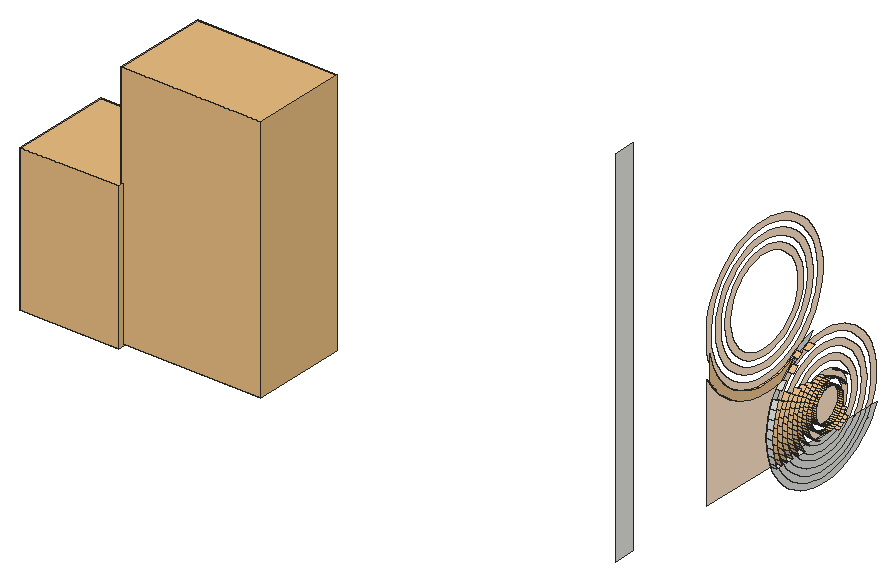
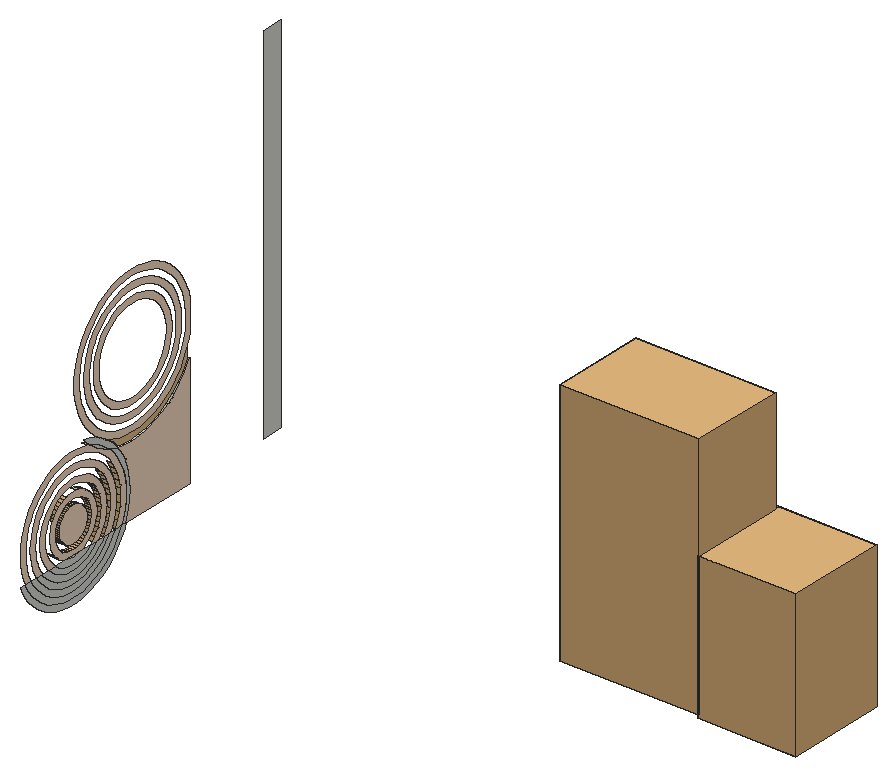
# SketchUp Ruby script. Lengths in inches.
U = 1.inch
M = Sketchup.active_model
def pt(a) = Geom::Point3d.new(a.map { |v| v * U })
def face(e, loops, mat)
  f = e.add_face(loops[0].map { |a| pt(a) })
  loops[1..].each { |l| e.add_face(l.map { |a| pt(a) }).erase! }
  f.material = f.back_material = mat if mat
  f
end
# faces: each face lists its corners as indices into pts; further lists are holes
def faces(e, pts, list, mat = nil) = list.each { |f| face(e, (f[0].is_a?(Array) ? f : [f]).map { |l| l.map { |i| pts[i] } }, mat) }
# xy, xz, yz: faces in a plane at the given z, y or x. An outline is a flat list of corners, or four numbers for a rectangle; further outlines are holes
def ring(l) = l.size == 4 ? [[l[0], l[1]], [l[2], l[1]], [l[2], l[3]], [l[0], l[3]]] : l.each_slice(2).to_a
def flat(e, list, mat, &to3) = list.each { |f| face(e, (f[0].is_a?(Array) ? f : [f]).map { |l| ring(l).map { |u, v| to3.(u, v) } }, mat) }
def xy(e, z, list, mat = nil) = flat(e, list, mat) { |x, y| [x, y, z] }
def xz(e, y, list, mat = nil) = flat(e, list, mat) { |x, z| [x, y, z] }
def yz(e, x, list, mat = nil) = flat(e, list, mat) { |y, z| [x, y, z] }
def lines(e, pts, list) = list.each { |a, b| e.add_line(pt(pts[a]), pt(pts[b])) }
# prism: a flat outline (further loops are holes) pulled along v
def prism(e, loops, v, mat = nil)
  f = face(e, loops, mat); d = Geom::Vector3d.new(v.map { |x| x * U })
  f.pushpull(f.normal.samedirection?(d) ? d.length : -d.length)
end
def box(e, o, s, mat = nil) = prism(e, [[o, [o[0] + s[0], o[1], o[2]], [o[0] + s[0], o[1] + s[1], o[2]], [o[0], o[1] + s[1], o[2]]]], [0, 0, s[2]], mat)
def at(x, y, z, deg = 0) = Geom::Transformation.translation(pt([x, y, z])) * Geom::Transformation.rotation(ORIGIN, Z_AXIS, deg.degrees)
def axes(o, x, y, z) = Geom::Transformation.new([*x, 0, *y, 0, *z, 0, *pt(o).to_a, 1])
def part(name) = M.definitions.add(name)
# library, detail: a bought-in or finely detailed component or shape, given as its bounding box
def library(name, o, s) = part(name).tap { |d| box(d.entities, o, s) }
def detail(e, o, s) = box(e.add_group.entities, o, s)
def put(e, d, t, mat = nil) = e.add_instance(d, t).tap { |i| i.material = mat if mat }
def group(e, t, mat = nil) = e.add_group.tap { |g| g.transformation = t; g.material = mat if mat }.entities
root = M.entities
M.materials.add("[Color C02]").color = [255, 228, 201]
M.materials.add("images").color = [235, 194, 141]
c1 = library("Group\#206",[0,0,0],[32.28,33.03,47.79])
c2 = library("Group\#215",[0,0,0],[15.67,22.625,14.53])
c3 = library("Group\#212",[0,0.16,0],[45.87,31.27,81.21])
xy(root,0,[[183.82,72.6875,185.82,74.8],[183.82,77.01,185.82,79.31],[183.82,81.7,185.82,84.26]])
xy(root,1.47,[[183.82,93.95,185.82,94.83]],"images")
xy(root,3.46,[[183.82,94.0625,185.82,94.72]],"images")
xy(root,14.7,[[183.82,94.0625,185.82,94.72]],"images")
xy(root,16.69,[[183.82,93.95,185.82,94.83]],"images")
yz(root,183.82,[[93.02,-14.45,95.76,-14.45,98.48,-14.125,101.15,-13.49,103.72,-12.56,106.17,-11.33,108.46,-9.82,110.5625,-8.0625,112.44,-6.07,114.08,-3.87,115.45,-1.5,116.09,0,113.98,0,113.71,-0.625,112.46,-2.8,110.96,-4.82,109.23,-6.65,107.3,-8.27,105.2,-9.65,102.96,-10.78,100.59,-11.64,98.14,-12.22,95.65,-12.51,93.13,-12.51,90.63,-12.22,88.1875,-11.64,85.82,-10.78,83.58,-9.65,81.48,-8.27,79.55,-6.65,77.82,-4.82,76.32,-2.8,75.06,-0.625,74.8,0,72.6875,0,73.33,-1.5,74.7,-3.87,76.34,-6.07,78.22,-8.0625,80.32,-9.82,82.61,-11.33,85.06,-12.56,87.63,-13.49,90.3,-14.125],[93.13,-12.51,95.65,-12.51,98.14,-12.22,100.59,-11.64,102.96,-10.78,105.2,-9.65,107.3,-8.27,109.23,-6.65,110.96,-4.82,112.46,-2.8,113.71,-0.625,113.98,0,111.77,0,110.79,-1.7,109.42,-3.53,107.86,-5.19,106.11,-6.66,104.2,-7.92,102.16,-8.94,100.02,-9.72,97.8,-10.25,95.53,-10.51,93.25,-10.51,90.98,-10.25,88.76,-9.72,86.62,-8.94,84.58,-7.92,82.67,-6.66,80.92,-5.19,79.36,-3.53,77.99,-1.7,77.01,0,74.8,0,75.06,-0.625,76.32,-2.8,77.82,-4.82,79.55,-6.65,81.48,-8.27,83.58,-9.65,85.82,-10.78,88.1875,-11.64,90.63,-12.22],[93.25,-10.51,95.53,-10.51,97.8,-10.25,100.02,-9.72,102.16,-8.94,104.2,-7.92,106.11,-6.66,107.86,-5.19,109.42,-3.53,110.79,-1.7,111.77,0,109.46,0,109.12,-0.61,107.89,-2.25,106.48,-3.74,104.91,-5.06,103.2,-6.18,101.37,-7.1,99.44,-7.8,97.45,-8.28,95.41,-8.52,93.36,-8.52,91.33,-8.28,89.33,-7.8,87.41,-7.1,85.58,-6.18,83.86,-5.06,82.29,-3.74,80.89,-2.25,79.66,-0.61,79.31,0,77.01,0,77.99,-1.7,79.36,-3.53,80.92,-5.19,82.67,-6.66,84.58,-7.92,86.62,-8.94,88.76,-9.72,90.98,-10.25],[93.36,-8.52,95.41,-8.52,97.45,-8.28,99.44,-7.8,101.37,-7.1,103.2,-6.18,104.91,-5.06,106.48,-3.74,107.89,-2.25,109.12,-0.61,109.46,0,107.08,0,106.36,-0.96,105.11,-2.29,103.72,-3.45,102.2,-4.45,100.58,-5.27,98.87,-5.89,97.1,-6.31,95.3,-6.52,93.48,-6.52,91.68,-6.31,89.91,-5.89,88.2,-5.27,86.58,-4.45,85.06,-3.45,83.67,-2.29,82.42,-0.96,81.7,0,79.31,0,79.66,-0.61,80.89,-2.25,82.29,-3.74,83.86,-5.06,85.58,-6.18,87.41,-7.1,89.33,-7.8,91.33,-8.28],[93.48,-6.52,95.3,-6.52,97.1,-6.31,98.87,-5.89,100.58,-5.27,102.2,-4.45,103.72,-3.45,105.11,-2.29,106.36,-0.96,107.08,0,104.52,0,103.74,-0.83,102.53,-1.85,101.2,-2.72,99.79,-3.43,98.3,-3.97,96.76,-4.34,95.18,-4.52,93.6,-4.52,92.02,-4.34,90.48,-3.97,88.99,-3.43,87.58,-2.72,86.25,-1.85,85.04,-0.83,84.26,0,81.7,0,82.42,-0.96,83.67,-2.29,85.06,-3.45,86.58,-4.45,88.2,-5.27,89.91,-5.89,91.68,-6.31],
  [93.6,-4.52,95.18,-4.52,96.76,-4.34,98.3,-3.97,99.79,-3.43,101.2,-2.72,102.53,-1.85,103.74,-0.83,104.52,0,101.625,0,101.33,-0.24,100.2,-0.99,98.99,-1.59,97.72,-2.06,96.41,-2.37,95.07,-2.53,93.71,-2.53,92.37,-2.37,91.06,-2.06,89.79,-1.59,88.58,-0.99,87.45,-0.24,87.16,0,84.26,0,85.04,-0.83,86.25,-1.85,87.58,-2.72,88.99,-3.43,90.48,-3.97,92.02,-4.34],[93.71,-2.53,95.07,-2.53,96.41,-2.37,97.72,-2.06,98.99,-1.59,100.2,-0.99,101.33,-0.24,101.625,0,97.54,0,97.15,-0.14,96.0625,-0.4,94.95,-0.53,93.83,-0.53,92.72,-0.4,91.63,-0.14,91.24,0,87.16,0,87.45,-0.24,88.58,-0.99,89.79,-1.59,91.06,-2.06,92.37,-2.37],[93.83,-0.53,94.95,-0.53,96.0625,-0.4,97.15,-0.14,97.54,0,91.24,0,91.63,-0.14,92.72,-0.4],[9,0,16,120],[72.6875,0,74.8,0,74.07,1.68,73.35,4.09,72.91,6.57,72.76,9.08,72.91,11.59,73.35,14.07,74.07,16.48,75.06,18.79,76.32,20.96,77.82,22.98,79.55,24.81,79.6,24.85,79.04,24.61,76.06,23.74,75.96,23.72,74.7,22.03,73.33,19.66,72.25,17.14,71.46,14.51,70.98,11.82,70.82,9.08,70.98,6.34,71.46,3.65,72.25,1.02],
  [75.96,23.72,76.06,23.74,79.04,24.61,79.6,24.85,81.48,26.43,83.58,27.81,85.82,28.9375,87.43,29.52,89.38,31.34,90.15,32.25,87.63,31.65,85.06,30.72,83.42,29.9,83.11,29.67,81.36,28.67,80.32,27.98,78.22,26.22,76.34,24.23],[79.6,24.85,81.9,25.83,84.6,27.37,87.11,29.22,87.43,29.52,85.82,28.9375,83.58,27.81,81.48,26.43],[81.36,28.67,83.11,29.67,83.42,29.9,82.61,29.49]])
yz(root,183.82,[[46.5625,0,72.6875,0,72.25,1.02,71.46,3.65,70.98,6.34,70.82,9.08,70.98,11.82,71.46,14.51,72.25,17.14,73.33,19.66,74.7,22.03,75.96,23.72,72.99,23.21,69.89,23.05,66.79,23.24,63.73,23.8,60.75,24.7,57.9,25.95,55.22,27.52,52.73,29.39,50.48,31.53,48.49,33.92,46.8,36.53,46.5625,37.01],[74.8,0,77.01,0,76.85,0.27,75.95,2.37,75.29,4.55,74.9,6.8,74.76,9.08,74.9,11.36,75.29,13.61,75.95,15.79,76.85,17.89,77.99,19.86,79.36,21.69,80.92,23.35,82.67,24.82,84.58,26.08,86.62,27.1,88.76,27.88,90.98,28.41,93.25,28.67,95.53,28.67,97.8,28.41,100.02,27.88,102.16,27.1,104.2,26.08,106.11,24.82,107.86,23.35,109.42,21.69,110.79,19.86,111.93,17.89,112.83,15.79,113.49,13.61,113.88,11.36,114.01,9.08,113.88,6.8,113.49,4.55,112.83,2.37,111.93,0.27,111.77,0,113.98,0,114.71,1.68,115.43,4.09,115.87,6.57,116.01,9.08,115.87,11.59,115.43,14.07,114.71,16.48,113.71,18.79,112.46,20.96,110.96,22.98,109.23,24.81,107.3,26.43,105.2,27.81,102.96,28.9375,100.59,29.8,98.14,30.375,95.65,30.67,93.13,30.67,90.63,30.375,88.1875,29.8,87.43,29.52,87.11,29.22,84.6,27.37,81.9,25.83,79.6,24.85,79.55,24.81,77.82,22.98,76.32,20.96,75.06,18.79,74.07,16.48,73.35,14.07,72.91,11.59,72.76,9.08,72.91,6.57,73.35,4.09,74.07,1.68],[79.31,0,81.7,0,81.34,0.49,80.43,2.07,79.71,3.74,79.1875,5.48,78.87,7.27,78.76,9.08,78.87,10.89,79.1875,12.68,79.71,14.42,80.43,16.09,81.34,17.67,82.42,19.125,83.67,20.45,85.06,21.61,86.58,22.61,88.2,23.43,89.91,24.05,91.68,24.47,93.48,24.68,95.3,24.68,97.1,24.47,98.87,24.05,100.58,23.43,102.2,22.61,103.72,21.61,105.11,20.45,106.36,19.125,107.44,17.67,108.35,16.09,109.07,14.42,109.59,12.68,109.91,10.89,110.01,9.08,109.91,7.27,109.59,5.48,109.07,3.74,108.35,2.07,107.44,0.49,107.08,0,109.46,0,110.14,1.17,110.95,3.05,111.54,5.02,111.9,7.03,112.01,9.08,111.9,11.125,111.54,13.14,110.95,15.11,110.14,16.99,109.12,18.77,107.89,20.41,106.48,21.9,104.91,23.22,103.2,24.34,101.37,25.26,99.44,25.96,97.45,26.4375,95.41,26.68,93.36,26.68,91.33,26.4375,89.33,25.96,87.41,25.26,85.58,24.34,83.86,23.22,82.29,21.9,80.89,20.41,79.66,18.77,78.64,16.99,77.83,15.11,77.24,13.14,76.88,11.125,76.76,9.08,76.88,7.03,77.24,5.02,77.83,3.05,78.64,1.17],[84.26,0,87.16,0,86.41,0.625,85.48,1.61,84.68,2.69,84,3.86,83.47,5.1,83.08,6.4,82.84,7.73,82.76,9.08,82.84,10.43,83.08,11.76,83.47,13.06,84,14.3,84.68,15.47,85.48,16.55,86.41,17.54,87.45,18.4,88.58,19.15,89.79,19.75,91.06,20.22,92.37,20.53,93.71,20.69,95.07,20.69,96.41,20.53,97.72,20.22,98.99,19.75,100.2,19.15,101.33,18.4,102.37,17.54,103.3,16.55,104.1,15.47,104.78,14.3,105.3125,13.06,105.7,11.76,105.9375,10.43,106.01,9.08,105.9375,7.73,105.7,6.4,105.3125,5.1,104.78,3.86,104.1,2.69,103.3,1.61,102.37,0.625,101.625,0,104.52,0,104.83,0.32,105.77,1.59,106.57,2.97,107.19,4.42,107.65,5.9375,107.92,7.5,108.01,9.08,107.92,10.66,107.65,12.22,107.19,13.74,106.57,15.19,105.77,16.57,104.83,17.84,103.74,18.99,102.53,20.01,101.2,20.88,99.79,21.59,98.3,22.13,96.76,22.5,95.18,22.68,93.6,22.68,92.02,22.5,90.48,22.13,88.99,21.59,87.58,20.88,86.25,20.01,85.04,18.99,83.95,17.84,83.01,16.57,82.21,15.19,81.59,13.74,81.13,12.22,80.86,10.66,80.76,9.08,80.86,7.5,81.13,5.9375,81.59,4.42,82.21,2.97,83.01,1.59,83.95,0.32],[[91.24,0,97.54,0,98.2,0.24,99.2,0.74,100.14,1.36,100.99,2.08,101.76,2.89,102.43,3.79,102.99,4.76,103.43,5.79,103.76,6.86,103.95,7.96,104.01,9.08,103.95,10.2,103.76,11.3,103.43,12.37,102.99,13.4,102.43,14.37,101.76,15.27,100.99,16.08,100.14,16.8,99.2,17.42,98.2,17.92,97.15,18.3,96.0625,18.56,94.95,18.6875,93.83,18.6875,92.72,18.56,91.63,18.3,90.58,17.92,89.58,17.42,88.64,16.8,87.78,16.08,87.02,15.27,86.35,14.37,85.79,13.4,85.35,12.37,85.02,11.3,84.83,10.2,84.76,9.08,84.83,7.96,85.02,6.86,85.35,5.79,85.79,4.76,86.35,3.79,87.02,2.89,87.78,2.08,88.64,1.36,89.58,0.74,90.58,0.24],[93.95,1.47,93.07,1.57,92.2,1.78,91.37,2.08,90.58,2.48,89.84,2.96,89.16,3.53,88.55,4.18,88.02,4.89,87.58,5.66,87.22,6.47,86.97,7.32,86.82,8.19,86.76,9.08,86.82,9.97,86.97,10.84,87.22,11.6875,87.58,12.5,88.02,13.27,88.55,13.98,89.16,14.625,89.84,15.2,90.58,15.68,91.37,16.08,92.2,16.38,93.07,16.59,93.95,16.69,94.83,16.69,95.71,16.59,96.58,16.38,97.41,16.08,98.2,15.68,98.94,15.2,99.62,14.625,100.23,13.98,100.76,13.27,101.2,12.5,101.55,11.6875,101.81,10.84,101.96,9.97,102.01,9.08,101.96,8.19,101.81,7.32,101.55,6.47,101.2,5.66,100.76,4.89,100.23,4.18,99.62,3.53,98.94,2.96,98.2,2.48,97.41,2.08,96.58,1.78,95.71,1.57,94.83,1.47]],
  [94.0625,3.46,94.72,3.46,95.37,3.54,96,3.69,96.62,3.92,97.2,4.21,97.75,4.57,98.25,4.99,98.7,5.46,99.09,5.99,99.42,6.56,99.68,7.16,99.86,7.78,99.98,8.43,100.01,9.08,99.98,9.73,99.86,10.38,99.68,11,99.42,11.6,99.09,12.17,98.7,12.7,98.25,13.17,97.75,13.59,97.2,13.95,96.62,14.24,96,14.47,95.37,14.62,94.72,14.7,94.0625,14.7,93.41,14.62,92.78,14.47,92.16,14.24,91.58,13.95,91.03,13.59,90.53,13.17,90.08,12.7,89.69,12.17,89.36,11.6,89.1,11,88.92,10.38,88.8,9.73,88.76,9.08,88.8,8.43,88.92,7.78,89.1,7.16,89.36,6.56,89.69,5.99,90.08,5.46,90.53,4.99,91.03,4.57,91.58,4.21,92.16,3.92,92.78,3.69,93.41,3.54],[[69.9,25.78,72.6875,25.93,75.44,26.4,78.12,27.19,80.6875,28.28,81.36,28.67,82.61,29.49,83.42,29.9,85.36,31.32,87.4,33.23,89.2,35.36,90.75,37.68,92.01,40.17,92.98,42.79,93.64,45.5,93.97,48.27,93.98,49.89,93.99,51.06,93.68,53.83,93.05,56.55,92.1,59.18,90.86,61.68,90.41,62.38,89.34,64.02,87.56,66.17,85.54,68.09,83.31,69.77,80.9,71.18,78.34,72.29,75.67,73.11,72.92,73.61,70.14,73.78,67.35,73.63,64.6,73.16,61.92,72.375,59.36,71.28,56.93,69.9,54.68,68.24,52.65,66.34,50.84,64.21,49.3,61.89,48.03,59.4,47.0625,56.78,46.5625,54.71,46.5625,44.88,47,43.01,47.9375,40.39,49.18,37.89,50.7,35.55,52.48,33.4,54.5,31.47,56.73,29.8,59.14,28.39,61.7,27.27,64.37,26.46,67.12,25.96],[69.91,27.78,67.36,27.94,64.84,28.4,62.39,29.15,60.05,30.17,57.84,31.46,55.8,33,53.94,34.76,52.31,36.73,50.91,38.88,49.78,41.17,48.91,43.58,48.34,46.07,48.05,48.61,48.0625,51.17,48.375,53.71,48.98,56.2,49.86,58.6,51.02,60.88,52.4375,63.01,54.09,64.96,55.96,66.71,58.02,68.22,60.24,69.49,62.6,70.49,65.05,71.21,67.57,71.65,70.13,71.78,72.68,71.62,75.2,71.16,77.65,70.42,79.99,69.39,82.2,68.1,84.25,66.57,86.1,64.8,87.73,62.83,89.13,60.6875,90.26,58.4,91.13,55.99,91.71,53.5,91.99,50.95,91.98,48.4,91.67,45.86,91.06,43.37,90.18,40.97,89.02,38.6875,87.6,36.56,85.95,34.61,84.08,32.86,82.02,31.34,79.8,30.07,77.44,29.07,74.99,28.35,72.47,27.92]],[[69.92,29.78,72.24,29.91,74.54,30.3,76.77,30.96,78.91,31.87,80.93,33.02,82.8,34.4,84.5,35.99,86,37.76,87.29,39.7,88.35,41.77,89.15,43.95,89.7,46.21,89.98,48.52,89.99,50.85,89.73,53.16,89.21,55.42,88.42,57.61,87.39,59.7,86.12,61.65,84.64,63.4375,82.95,65.04,81.09,66.4375,79.08,67.61,76.95,68.54,74.73,69.22,72.44,69.64,70.12,69.78,67.8,69.66,65.5,69.27,63.27,68.61,61.13,67.7,59.11,66.55,57.24,65.17,55.54,63.58,54.04,61.81,52.75,59.87,51.7,57.8,50.89,55.61,50.34,53.35,50.06,51.04,50.05,48.72,50.31,46.41,50.83,44.14,51.62,41.95,52.65,39.87,53.92,37.92,55.41,36.13,57.09,34.53,58.95,33.13,60.96,31.95,63.09,31.02,65.3125,30.35,67.6,29.93],[69.93,31.78,67.84,31.92,65.78,32.29,63.78,32.9,61.86,33.74,60.06,34.79,58.38,36.05,56.87,37.5,55.53,39.11,54.39,40.86,53.46,42.74,52.75,44.71,52.28,46.75,52.05,48.83,52.06,50.92,52.31,53,52.8,55.03,53.53,56.99,54.48,58.86,55.64,60.6,56.99,62.2,58.52,63.63,60.2,64.87,62.02,65.91,63.95,66.73,65.96,67.32,68.02,67.67,70.11,67.78,72.2,67.65,74.26,67.28,76.26,66.67,78.18,65.83,79.99,64.77,81.66,63.51,83.17,62.07,84.51,60.46,85.65,58.71,86.58,56.83,87.29,54.86,87.76,52.82,88,50.74,87.98,48.65,87.73,46.57,87.24,44.54,86.51,42.57,85.5625,40.71,84.41,38.96,83.05,37.37,81.52,35.9375,79.84,34.7,78.02,33.66,76.09,32.84,74.09,32.25,72.02,31.89]],[[69.94,33.78,71.8,33.88,73.63,34.2,75.42,34.72,77.13,35.45,78.75,36.37,80.24,37.48,81.6,38.75,82.81,40.17,83.84,41.71,84.68,43.375,85.33,45.12,85.76,46.93,85.99,48.77,86,50.63,85.79,52.48,85.37,54.3,84.74,56.05,83.92,57.71,82.9,59.27,81.71,60.71,80.37,61.99,78.88,63.11,77.27,64.05,75.57,64.79,73.79,65.33,71.96,65.67,70.1,65.78,68.24,65.68,66.41,65.37,64.62,64.84,62.91,64.12,61.29,63.19,59.8,62.09,58.4375,60.82,57.23,59.4,56.2,57.85,55.36,56.19,54.72,54.45,54.28,52.64,54.05,50.79,54.04,48.93,54.25,47.08,54.67,45.27,55.3,43.52,56.125,41.85,57.14,40.29,58.33,38.86,59.68,37.58,61.16,36.46,62.77,35.52,64.47,34.78,66.25,34.23,68.08,33.9],[69.95,35.78,68.33,35.89,66.72,36.18,65.17,36.65,63.68,37.3,62.27,38.125,60.97,39.1,59.79,40.23,58.75,41.48,57.86,42.84,57.14,44.3,56.59,45.83,56.22,47.42,56.04,49.04,56.05,50.67,56.25,52.28,56.63,53.86,57.19,55.39,57.93,56.84,58.83,58.2,59.88,59.44,61.07,60.55,62.39,61.52,63.8,62.32,65.3,62.96,66.86,63.42,68.46,63.7,70.09,63.78,71.71,63.68,73.32,63.39,74.875,62.91,76.37,62.26,77.77,61.44,79.07,60.46,80.25,59.34,81.29,58.09,82.18,56.72,82.9,55.26,83.45,53.73,83.82,52.15,84,50.53,83.99,48.9,83.8,47.28,83.41,45.7,82.85,44.17,82.11,42.72,81.21,41.37,80.16,40.125,78.97,39.01,77.66,38.05,76.24,37.24,74.74,36.6,73.18,36.14,71.58,35.87]]],"[Color C02]")
yz(root,184.63,[[69.89,23.05,72.99,23.21,75.96,23.72,76.34,24.23,78.22,26.22,80.32,27.98,81.36,28.67,80.6875,28.28,78.12,27.19,75.44,26.4,72.6875,25.93,69.9,25.78,67.12,25.96,64.37,26.46,61.7,27.27,59.14,28.39,56.73,29.8,54.5,31.47,52.48,33.4,50.7,35.55,49.18,37.89,47.9375,40.39,47,43.01,46.5625,44.88,46.5625,37.01,46.8,36.53,48.49,33.92,50.48,31.53,52.73,29.39,55.22,27.52,57.9,25.95,60.75,24.7,63.73,23.8,66.79,23.24]],"images")
p = [[183.82,72.25,1.02],[183.82,72.6875,0],[185.82,72.6875,0],[185.82,72.25,1.02],[183.82,74.8,0],[183.82,74.07,1.68],
  [185.82,74.07,1.68],[185.82,74.8,0],[183.82,76.85,0.27],[183.82,77.01,0],[185.82,77.01,0],[185.82,76.85,0.27],
  [183.82,79.31,0],[183.82,78.64,1.17],[185.82,78.64,1.17],[185.82,79.31,0],[183.82,81.34,0.49],[183.82,81.7,0],
  [185.82,81.7,0],[185.82,81.34,0.49],[183.82,84.26,0],[183.82,83.95,0.32],[185.82,83.95,0.32],[185.82,84.26,0],
  [183.82,90.58,0.24],[183.82,89.58,0.74],[185.82,89.58,0.74],[185.82,90.58,0.24],[183.82,99.2,0.74],[183.82,98.2,0.24],
  [185.82,98.2,0.24],[185.82,99.2,0.74],[183.82,75.95,2.37],[185.82,75.95,2.37],[183.82,83.01,1.59],[185.82,83.01,1.59],
  [183.82,80.43,2.07],[185.82,80.43,2.07],[183.82,85.48,1.61],[183.82,86.41,0.625],[185.82,86.41,0.625],[185.82,85.48,1.61],
  [183.82,88.64,1.36],[185.82,88.64,1.36],[183.82,100.14,1.36],[185.82,100.14,1.36],[183.82,71.46,3.65],[185.82,71.46,3.65],
  [183.82,77.83,3.05],[185.82,77.83,3.05],[183.82,87.78,2.08],[185.82,87.78,2.08],[183.82,100.99,2.08],[185.82,100.99,2.08],
  [183.82,93.07,1.57],[183.82,93.95,1.47],[185.82,93.95,1.47],[185.82,93.07,1.57],[183.82,94.83,1.47],[183.82,95.71,1.57],
  [185.82,95.71,1.57],[185.82,94.83,1.47],[183.82,82.21,2.97],[185.82,82.21,2.97],[183.82,84.68,2.69],[185.82,84.68,2.69],
  [183.82,92.2,1.78],[185.82,92.2,1.78],[183.82,96.58,1.78],[185.82,96.58,1.78],[183.82,73.35,4.09],[185.82,73.35,4.09],
  [183.82,91.37,2.08],[185.82,91.37,2.08],[183.82,97.41,2.08],[185.82,97.41,2.08],[183.82,79.71,3.74],[185.82,79.71,3.74],
  [183.82,87.02,2.89],[185.82,87.02,2.89],[183.82,90.58,2.48],[185.82,90.58,2.48],[183.82,98.2,2.48],[185.82,98.2,2.48],
  [183.82,101.76,2.89],[185.82,101.76,2.89],[183.82,75.29,4.55],[185.82,75.29,4.55],[183.82,89.84,2.96],[185.82,89.84,2.96],
  [183.82,98.94,2.96],[185.82,98.94,2.96],[183.82,84,3.86],[185.82,84,3.86],[183.82,86.35,3.79],[185.82,86.35,3.79],
  [183.82,81.59,4.42],[185.82,81.59,4.42],[183.82,89.16,3.53],[185.82,89.16,3.53],[183.82,99.62,3.53],[185.82,99.62,3.53],
  [183.82,77.24,5.02],[185.82,77.24,5.02],[183.82,88.55,4.18],[185.82,88.55,4.18],[183.82,93.41,3.54],[183.82,92.78,3.69],
  [185.82,92.78,3.69],[185.82,93.41,3.54],[183.82,94.0625,3.46],[185.82,94.0625,3.46],[183.82,95.37,3.54],[183.82,94.72,3.46],
  [185.82,94.72,3.46],[185.82,95.37,3.54],[183.82,96,3.69],[185.82,96,3.69],[183.82,100.23,4.18],[185.82,100.23,4.18],
  [183.82,70.98,6.34],[185.82,70.98,6.34],[183.82,79.1875,5.48],[185.82,79.1875,5.48],[183.82,92.16,3.92],[185.82,92.16,3.92],
  [183.82,96.62,3.92],[185.82,96.62,3.92],[183.82,85.79,4.76],[185.82,85.79,4.76],[183.82,83.47,5.1],[185.82,83.47,5.1],
  [183.82,91.58,4.21],[185.82,91.58,4.21],[183.82,97.2,4.21],[185.82,97.2,4.21],[183.82,72.91,6.57],[185.82,72.91,6.57],
  [183.82,88.02,4.89],[185.82,88.02,4.89],[183.82,91.03,4.57],[185.82,91.03,4.57],[183.82,97.75,4.57],[185.82,97.75,4.57],
  [183.82,100.76,4.89],[185.82,100.76,4.89],[183.82,81.13,5.9375],[185.82,81.13,5.9375],[183.82,74.9,6.8],[185.82,74.9,6.8],
  [183.82,90.53,4.99],[185.82,90.53,4.99],[183.82,98.25,4.99],[185.82,98.25,4.99],[183.82,85.35,5.79],[185.82,85.35,5.79],
  [183.82,87.58,5.66],[185.82,87.58,5.66],[183.82,101.2,5.66],[185.82,101.2,5.66],[183.82,76.88,7.03],[185.82,76.88,7.03],
  [183.82,90.08,5.46],[185.82,90.08,5.46],[183.82,98.7,5.46],[185.82,98.7,5.46],[183.82,83.08,6.4],[185.82,83.08,6.4],
  [183.82,78.87,7.27],[185.82,78.87,7.27],[183.82,89.69,5.99],[185.82,89.69,5.99],[183.82,99.09,5.99],[185.82,99.09,5.99],
  [183.82,87.22,6.47],[185.82,87.22,6.47],[183.82,85.02,6.86],[185.82,85.02,6.86],[183.82,80.86,7.5],[185.82,80.86,7.5],
  [183.82,89.36,6.56],[185.82,89.36,6.56],[183.82,99.42,6.56],[185.82,99.42,6.56],[183.82,70.82,9.08],[185.82,70.82,9.08],
  [183.82,82.84,7.73],[185.82,82.84,7.73],[183.82,86.97,7.32],[185.82,86.97,7.32],[183.82,72.76,9.08],[185.82,72.76,9.08],
  [183.82,89.1,7.16],[185.82,89.1,7.16],[183.82,99.68,7.16],[185.82,99.68,7.16],[183.82,74.76,9.08],[185.82,74.76,9.08],
  [183.82,84.83,7.96],[185.82,84.83,7.96],[183.82,76.76,9.08],[185.82,76.76,9.08],[183.82,88.92,7.78],[185.82,88.92,7.78],
  [183.82,99.86,7.78],[185.82,99.86,7.78],[183.82,78.76,9.08],[185.82,78.76,9.08],[183.82,86.82,8.19],[185.82,86.82,8.19],
  [183.82,80.76,9.08],[185.82,80.76,9.08],[183.82,82.76,9.08],[185.82,82.76,9.08],[183.82,88.8,8.43],[185.82,88.8,8.43],
  [183.82,99.98,8.43],[185.82,99.98,8.43],[183.82,84.76,9.08],[185.82,84.76,9.08],[183.82,86.76,9.08],[185.82,86.76,9.08],
  [183.82,88.76,9.08],[185.82,88.76,9.08],[183.82,100.01,9.08],[185.82,100.01,9.08],[183.82,70.98,11.82],[185.82,70.98,11.82],
  [183.82,72.91,11.59],[185.82,72.91,11.59],[183.82,74.9,11.36],[185.82,74.9,11.36],[183.82,76.88,11.125],[185.82,76.88,11.125],
  [183.82,78.87,10.89],[185.82,78.87,10.89],[183.82,80.86,10.66],[185.82,80.86,10.66],[183.82,82.84,10.43],[185.82,82.84,10.43],
  [183.82,84.83,10.2],[185.82,84.83,10.2],[183.82,86.82,9.97],[185.82,86.82,9.97],[183.82,88.8,9.73],[185.82,88.8,9.73],
  [183.82,99.98,9.73],[185.82,99.98,9.73],[183.82,88.92,10.38],[185.82,88.92,10.38],[183.82,99.86,10.38],[185.82,99.86,10.38],
  [183.82,86.97,10.84],[185.82,86.97,10.84],[183.82,85.02,11.3],[185.82,85.02,11.3],[183.82,83.08,11.76],[185.82,83.08,11.76],
  [183.82,89.1,11],[185.82,89.1,11],[183.82,99.68,11],[185.82,99.68,11],[183.82,81.13,12.22],[185.82,81.13,12.22],
  [183.82,87.22,11.6875],[185.82,87.22,11.6875],[183.82,79.1875,12.68],[185.82,79.1875,12.68],[183.82,89.36,11.6],[185.82,89.36,11.6],
  [183.82,99.42,11.6],[185.82,99.42,11.6],[183.82,77.24,13.14],[185.82,77.24,13.14],[183.82,85.35,12.37],[185.82,85.35,12.37],
  [183.82,75.29,13.61],[185.82,75.29,13.61],[183.82,73.35,14.07],[185.82,73.35,14.07],[183.82,89.69,12.17],[185.82,89.69,12.17],
  [183.82,99.09,12.17],[185.82,99.09,12.17],[183.82,87.58,12.5],[185.82,87.58,12.5],[183.82,71.46,14.51],[185.82,71.46,14.51],
  [183.82,83.47,13.06],[185.82,83.47,13.06],[183.82,81.59,13.74],[185.82,81.59,13.74],[183.82,90.08,12.7],[185.82,90.08,12.7],
  [183.82,98.7,12.7],[185.82,98.7,12.7],[183.82,85.79,13.4],[185.82,85.79,13.4],[183.82,88.02,13.27],[185.82,88.02,13.27],
  [183.82,101.2,12.5],[183.82,100.76,13.27],[185.82,100.76,13.27],[185.82,101.2,12.5],[183.82,79.71,14.42],[185.82,79.71,14.42],
  [183.82,90.53,13.17],[185.82,90.53,13.17],[183.82,98.25,13.17],[185.82,98.25,13.17],[183.82,77.83,15.11],[185.82,77.83,15.11],
  [183.82,84,14.3],[185.82,84,14.3],[183.82,91.03,13.59],[185.82,91.03,13.59],[183.82,97.75,13.59],[185.82,97.75,13.59],
  [183.82,88.55,13.98],[185.82,88.55,13.98],[183.82,100.23,13.98],[185.82,100.23,13.98],[183.82,86.35,14.37],[185.82,86.35,14.37],
  [183.82,75.95,15.79],[185.82,75.95,15.79],[183.82,91.58,13.95],[185.82,91.58,13.95],[183.82,97.2,13.95],[185.82,97.2,13.95],
  [183.82,82.21,15.19],[185.82,82.21,15.19],[183.82,89.16,14.625],[185.82,89.16,14.625],[183.82,92.16,14.24],[185.82,92.16,14.24],
  [183.82,96.62,14.24],[185.82,96.62,14.24],[183.82,99.62,14.625],[185.82,99.62,14.625],[183.82,74.07,16.48],[185.82,74.07,16.48],
  [183.82,92.78,14.47],[185.82,92.78,14.47],[183.82,96,14.47],[185.82,96,14.47],[183.82,84.68,15.47],[185.82,84.68,15.47],
  [183.82,80.43,16.09],[185.82,80.43,16.09],[183.82,87.02,15.27],[185.82,87.02,15.27],[183.82,72.25,17.14],[185.82,72.25,17.14],
  [183.82,93.41,14.62],[185.82,93.41,14.62],[183.82,95.37,14.62],[185.82,95.37,14.62],[183.82,89.84,15.2],[185.82,89.84,15.2],
  [183.82,94.0625,14.7],[185.82,94.0625,14.7],[183.82,94.72,14.7],[185.82,94.72,14.7],[183.82,98.94,15.2],[185.82,98.94,15.2],
  [183.82,78.64,16.99],[185.82,78.64,16.99],[183.82,83.01,16.57],[185.82,83.01,16.57],[183.82,90.58,15.68],[185.82,90.58,15.68],
  [183.82,98.2,15.68],[185.82,98.2,15.68],[183.82,87.78,16.08],[185.82,87.78,16.08],[183.82,100.99,16.08],[183.82,101.76,15.27],
  [185.82,101.76,15.27],[185.82,100.99,16.08],[183.82,85.48,16.55],[185.82,85.48,16.55],[183.82,91.37,16.08],[185.82,91.37,16.08],
  [183.82,97.41,16.08],[185.82,97.41,16.08],[183.82,76.85,17.89],[185.82,76.85,17.89],[183.82,81.34,17.67],[185.82,81.34,17.67],
  [183.82,88.64,16.8],[185.82,88.64,16.8],[183.82,92.2,16.38],[185.82,92.2,16.38],[183.82,96.58,16.38],[185.82,96.58,16.38],
  [183.82,100.14,16.8],[185.82,100.14,16.8],[183.82,93.07,16.59],[185.82,93.07,16.59],[183.82,95.71,16.59],[185.82,95.71,16.59],
  [183.82,75.06,18.79],[185.82,75.06,18.79],[183.82,83.95,17.84],[185.82,83.95,17.84],[183.82,86.41,17.54],[185.82,86.41,17.54],
  [183.82,93.95,16.69],[185.82,93.95,16.69],[183.82,94.83,16.69],[185.82,94.83,16.69],[183.82,89.58,17.42],[185.82,89.58,17.42],
  [183.82,99.2,17.42],[185.82,99.2,17.42],[183.82,79.66,18.77],[185.82,79.66,18.77],[183.82,73.33,19.66],[185.82,73.33,19.66],
  [183.82,90.58,17.92],[185.82,90.58,17.92],[183.82,98.2,17.92],[185.82,98.2,17.92],[183.82,87.45,18.4],[185.82,87.45,18.4],
  [183.82,82.42,19.125],[185.82,82.42,19.125],[183.82,85.04,18.99],[185.82,85.04,18.99],[183.82,77.99,19.86],[185.82,77.99,19.86],
  [183.82,91.63,18.3],[185.82,91.63,18.3],[183.82,97.15,18.3],[185.82,97.15,18.3],[183.82,92.72,18.56],[185.82,92.72,18.56],
  [183.82,75.96,23.72],[183.82,74.7,22.03],[185.82,74.7,22.03],[185.82,76.34,24.23],[184.63,76.34,24.23],[184.63,75.96,23.72],
  [183.82,66.79,23.24],[183.82,69.89,23.05],[184.63,69.89,23.05],[184.63,66.79,23.24],[183.82,72.99,23.21],[184.63,72.99,23.21],
  [183.82,63.73,23.8],[184.63,63.73,23.8],[183.82,76.34,24.23],[183.82,60.75,24.7],[184.63,60.75,24.7],[183.82,78.22,26.22],
  [184.63,78.22,26.22],[183.82,57.9,25.95],[184.63,57.9,25.95],[183.82,79.55,24.81],[183.82,79.6,24.85],[183.82,81.48,26.43],
  [185.82,81.48,26.43],[185.82,79.55,24.81],[183.82,69.9,25.78],[183.82,67.12,25.96],[184.63,67.12,25.96],[184.63,69.9,25.78],
  [183.82,72.6875,25.93],[184.63,72.6875,25.93],[183.82,55.22,27.52],[184.63,55.22,27.52],[183.82,75.44,26.4],[184.63,75.44,26.4],
  [183.82,64.37,26.46],[184.63,64.37,26.46],[183.82,80.32,27.98],[184.63,80.32,27.98],[183.82,78.12,27.19],[184.63,78.12,27.19],
  [183.82,61.7,27.27],[184.63,61.7,27.27],[183.82,80.6875,28.28],[184.63,80.6875,28.28],[183.82,59.14,28.39],[184.63,59.14,28.39],
  [183.82,52.73,29.39],[184.63,52.73,29.39],[183.82,81.36,28.67],[184.63,81.36,28.67],[183.82,56.73,29.8],[184.63,56.73,29.8],
  [183.82,83.11,29.67],[185.82,81.36,28.67],[185.82,83.11,29.67],[183.82,85.82,28.9375],[183.82,87.43,29.52],[183.82,88.1875,29.8],
  [185.82,88.1875,29.8],[185.82,85.82,28.9375],[183.82,50.48,31.53],[184.63,50.48,31.53],[183.82,54.5,31.47],[184.63,54.5,31.47],
  [183.82,48.49,33.92],[184.63,48.49,33.92],[183.82,52.48,33.4],[184.63,52.48,33.4],[183.82,50.7,35.55],[184.63,50.7,35.55],
  [183.82,46.8,36.53],[184.63,46.8,36.53],[183.82,49.18,37.89],[184.63,49.18,37.89],[183.82,46.5625,37.01],[184.63,46.5625,37.01]]
faces(root,p,[[0,1,2,3],[46,0,3,47],[120,46,47,121],[184,120,121,185],[226,184,185,227],[286,226,227,287],[352,286,287,353],[418,352,353,419],
  [438,439,440,441,442,443],[444,445,446,447],[445,448,449,446],[450,444,447,451],[448,438,443,449],[452,438,443,442],[453,450,451,454],[455,452,442,456],
  [457,453,454,458],[470,457,458,471],[476,455,456,477],[486,470,471,487],[488,476,477,489],[500,486,487,501],[504,500,501,505],[510,504,505,511],
  [514,510,511,515]])
faces(root,p,[[4,5,6,7],[8,9,10,11],[12,13,14,15],[16,17,18,19],[20,21,22,23],[24,25,26,27],[28,29,30,31],[32,8,11,33],
  [21,34,35,22],[36,16,19,37],[38,39,40,41],[25,42,43,26],[44,28,31,45],[13,48,49,14],[42,50,51,43],[52,44,45,53],
  [54,55,56,57],[58,59,60,61],[34,62,63,35],[64,38,41,65],[66,54,57,67],[59,68,69,60],[5,70,71,6],[72,66,67,73],
  [68,74,75,69],[76,36,37,77],[50,78,79,51],[80,72,73,81],[74,82,83,75],[84,52,53,85],[86,32,33,87],[88,80,81,89],
  [82,90,91,83],[92,64,65,93],[78,94,95,79],[62,96,97,63],[98,88,89,99],[90,100,101,91],[48,102,103,49],[104,98,99,105],
  [106,107,108,109],[110,106,109,111],[112,113,114,115],[116,112,115,117],[100,118,119,101],[122,76,77,123],[107,124,125,108],[126,116,117,127],
  [94,128,129,95],[130,92,93,131],[124,132,133,125],[134,126,127,135],[70,136,137,71],[138,104,105,139],[132,140,141,133],[142,134,135,143],
  [118,144,145,119],[96,146,147,97],[148,86,87,149],[140,150,151,141],[152,142,143,153],[128,154,155,129],[156,138,139,157],[144,158,159,145],
  [102,160,161,103],[150,162,163,151],[164,152,153,165],[166,130,131,167],[168,122,123,169],[162,170,171,163],[172,164,165,173],[174,156,157,175],
  [154,176,177,155],[146,178,179,147],[170,180,181,171],[182,172,173,183],[186,166,167,187],[188,174,175,189],[136,190,191,137],[180,192,193,181],
  [194,182,183,195],[196,148,149,197],[176,198,199,177],[160,200,201,161],[192,202,203,193],[204,194,195,205],[206,168,169,207],[208,188,189,209],
  [178,210,211,179],[212,186,187,213],[202,214,215,203],[216,204,205,217],[198,218,219,199],[220,208,209,221],[214,222,223,215],[224,216,217,225],
  [190,228,229,191],[230,196,197,231],[200,232,233,201],[234,206,207,235],[210,236,237,211],[238,212,213,239],[218,240,241,219],[242,220,221,243],
  [222,244,245,223],[246,224,225,247],[244,248,249,245],[250,246,247,251],[252,242,243,253],[240,254,255,241],[256,238,239,257],[248,258,259,249],
  [260,250,251,261],[236,262,263,237],[264,252,253,265],[266,234,235,267],[258,268,269,259],[270,260,261,271],[232,272,273,233],[254,274,275,255],
  [276,230,231,277],[228,278,279,229],[268,280,281,269],[282,270,271,283],[284,264,265,285],[288,256,257,289],[262,290,291,263],[280,292,293,281],
  [294,282,283,295],[274,296,297,275],[298,284,285,299],[300,301,302,303],[304,266,267,305],[292,306,307,293],[308,294,295,309],[272,310,311,273],
  [312,288,289,313],[306,314,315,307],[316,308,309,317],[318,298,299,319],[301,320,321,302],[296,322,323,297],[324,276,277,325],[314,326,327,315],
  [328,316,317,329],[290,330,331,291],[332,318,319,333],[326,334,335,327],[336,328,329,337],[320,338,339,321],[278,340,341,279],[334,342,343,335],
  [344,336,337,345],[346,312,313,347],[348,304,305,349],[322,350,351,323],[342,354,355,343],[356,344,345,357],[358,332,333,359],[354,360,361,355],
  [362,356,357,363],[338,364,365,339],[310,366,367,311],[330,368,369,331],[370,358,359,371],[364,372,373,365],[350,374,375,351],[376,377,378,379],
  [380,346,347,381],[382,370,371,383],[372,384,385,373],[386,324,325,387],[388,348,349,389],[374,390,391,375],[392,382,383,393],[384,394,395,385],
  [396,376,379,397],[398,392,393,399],[394,400,401,395],[340,402,403,341],[368,404,405,369],[406,380,381,407],[408,398,399,409],[400,410,411,401],
  [390,412,413,391],[414,396,397,415],[366,416,417,367],[412,420,421,413],[422,414,415,423],[424,406,407,425],[426,388,389,427],[404,428,429,405],
  [430,386,387,431],[420,432,433,421],[434,422,423,435],[432,436,437,433],[459,460,461,462,463],[464,465,466,467],[468,464,467,469],[472,468,469,473],
  [465,474,475,466],[478,472,473,479],[474,480,481,475],[482,478,479,483],[480,484,485,481],[488,482,483,489],[484,490,491,485],[492,488,489,493,494],
  [495,496,497,498,499],[490,502,503,491],[502,506,507,503],[506,508,509,507],[508,512,513,509]],"images")
put(root,c1,at(-22.1,22.05,-4.08))
put(root,c2,at(6.5,31.05,28.74,90))
put(root,c3,at(9.79,23.47,-3.25))
